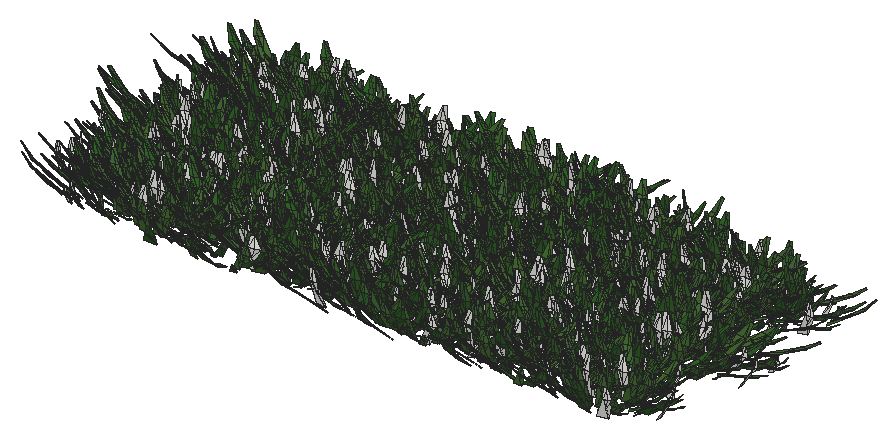
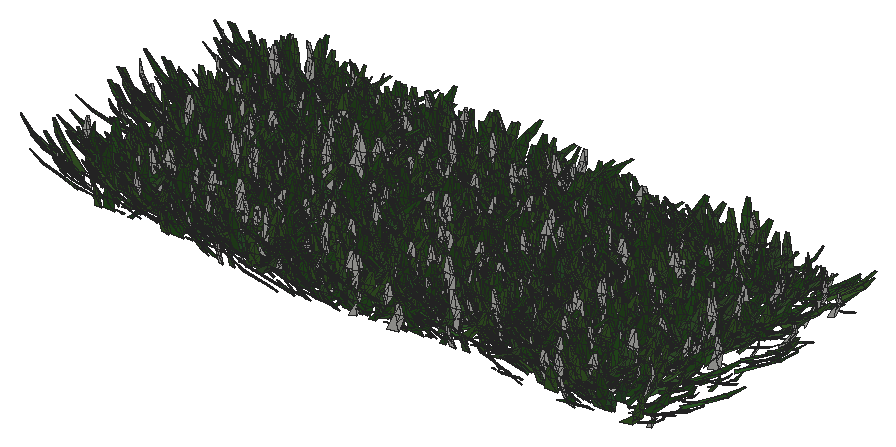
# SketchUp Ruby script. Lengths in inches.
U = 1.inch
M = Sketchup.active_model
def pt(a) = Geom::Point3d.new(a.map { |v| v * U })
def face(e, loops, mat)
  f = e.add_face(loops[0].map { |a| pt(a) })
  loops[1..].each { |l| e.add_face(l.map { |a| pt(a) }).erase! }
  f.material = f.back_material = mat if mat
  f
end
# faces: each face lists its corners as indices into pts; further lists are holes
def faces(e, pts, list, mat = nil) = list.each { |f| face(e, (f[0].is_a?(Array) ? f : [f]).map { |l| l.map { |i| pts[i] } }, mat) }
# xy, xz, yz: faces in a plane at the given z, y or x. An outline is a flat list of corners, or four numbers for a rectangle; further outlines are holes
def ring(l) = l.size == 4 ? [[l[0], l[1]], [l[2], l[1]], [l[2], l[3]], [l[0], l[3]]] : l.each_slice(2).to_a
def flat(e, list, mat, &to3) = list.each { |f| face(e, (f[0].is_a?(Array) ? f : [f]).map { |l| ring(l).map { |u, v| to3.(u, v) } }, mat) }
def xy(e, z, list, mat = nil) = flat(e, list, mat) { |x, y| [x, y, z] }
def xz(e, y, list, mat = nil) = flat(e, list, mat) { |x, z| [x, y, z] }
def yz(e, x, list, mat = nil) = flat(e, list, mat) { |y, z| [x, y, z] }
def lines(e, pts, list) = list.each { |a, b| e.add_line(pt(pts[a]), pt(pts[b])) }
# prism: a flat outline (further loops are holes) pulled along v
def prism(e, loops, v, mat = nil)
  f = face(e, loops, mat); d = Geom::Vector3d.new(v.map { |x| x * U })
  f.pushpull(f.normal.samedirection?(d) ? d.length : -d.length)
end
def box(e, o, s, mat = nil) = prism(e, [[o, [o[0] + s[0], o[1], o[2]], [o[0] + s[0], o[1] + s[1], o[2]], [o[0], o[1] + s[1], o[2]]]], [0, 0, s[2]], mat)
def at(x, y, z, deg = 0) = Geom::Transformation.translation(pt([x, y, z])) * Geom::Transformation.rotation(ORIGIN, Z_AXIS, deg.degrees)
def axes(o, x, y, z) = Geom::Transformation.new([*x, 0, *y, 0, *z, 0, *pt(o).to_a, 1])
def part(name) = M.definitions.add(name)
# library, detail: a bought-in or finely detailed component or shape, given as its bounding box
def library(name, o, s) = part(name).tap { |d| box(d.entities, o, s) }
def detail(e, o, s) = box(e.add_group.entities, o, s)
def put(e, d, t, mat = nil) = e.add_instance(d, t).tap { |i| i.material = mat if mat }
def group(e, t, mat = nil) = e.add_group.tap { |g| g.transformation = t; g.material = mat if mat }.entities
root = M.entities
M.materials.add("Material82").color = [68, 110, 58]
M.materials.add("Material83").color = [48, 90, 38]
M.materials.add("Material84").color = [68, 110, 48]
M.materials.add("Material85").color = [48, 90, 48]
M.materials.add("Material86").color = [58, 110, 58]
M.materials.add("Material87").color = [58, 90, 38]
M.materials.add("Material88").color = [68, 100, 58]
M.materials.add("Material89").color = [48, 100, 38]
c1 = part("grass00")
p = [[-0.6875,0.15,0],[-0.56,0.08,5.52],[-0.04,0.03,2.76],[0.48,-0.02,0],[0.35,-0.02,5.52],[-0.1,-0.14,5.52],
  [-0.12,0.65,8.37],[-0.42,0.65,8.37]]
faces(c1.entities,p,[[0,1,2,3],[3,2,4],[1,5,2],[5,4,2],[1,6,5],[4,5,6],[7,6,1]])
c2 = part("Group16\#1")
put(c2.entities,c1,axes([1.44,-0.61,-0.01],[0.05352,0.12609,0],[-0.10704,0.04543,0.07239],[0.06664,-0.02828,0.11628]),"Material85")
put(c2.entities,c1,axes([0.76,-0.15,-0.01],[0.04676,0.24062,0],[-0.23162,0.04501,0.06642],[0.0652,-0.01267,0.23595]),"Material82")
put(c2.entities,c1,axes([0.79,0.01,-0.01],[-0.00606,0.34651,0],[-0.34381,-0.00602,0.0432],[0.04319,0.00076,0.34386]))
put(c2.entities,c1,axes([1,0.23,-0.01],[-0.07192,0.31144,0],[-0.28722,-0.06632,0.1236],[0.12043,0.02781,0.29478]),"Material84")
put(c2.entities,c1,axes([1.66,0.77,-0.01],[-0.13828,0.29651,0],[-0.21551,-0.1005,0.22471],[0.20365,0.09498,0.23779]),"Material89")
put(c2.entities,c1,axes([0.6875,0.52,-0.01],[-0.18126,0.24051,0],[-0.22746,-0.17142,0.09788],[0.07817,0.05891,0.28481]),"Material84")
put(c2.entities,c1,axes([0.68,0.78,-0.01],[-0.215,0.18688,0],[-0.12385,-0.14248,0.21334],[0.13995,0.16101,0.18878]),"Material82")
put(c2.entities,c1,axes([0.56,1,-0.01],[-0.13756,0.07624,0],[-0.06159,-0.11112,0.0927],[0.04494,0.08108,0.12705]),"Material84")
put(c2.entities,c1,axes([0.2,0.64,-0.01],[-0.23729,0.07254,0],[-0.05711,-0.18681,0.153],[0.04473,0.14632,0.19535]),"Material89")
put(c2.entities,c1,axes([0.0625,0.72,-0.01],[-0.28874,0.02525,0],[-0.02179,-0.24916,0.14647],[0.01276,0.14591,0.25012]),"Material82")
put(c2.entities,c1,axes([-0.08,0.62,-0.01],[-0.34089,-0.04187,0],[0.03255,-0.26504,0.216],[-0.02633,0.21439,0.26703]),"Material89")
put(c2.entities,c1,axes([-0.34,0.98,-0.01],[-0.14314,-0.0493,0],[0.04397,-0.12769,0.06843],[-0.02228,0.0647,0.13505]),"Material89")
put(c2.entities,c1,axes([-0.87,1.45,-0.01],[-0.23488,-0.14114,0],[0.13761,-0.22901,0.06087],[-0.03135,0.05217,0.26717]))
put(c2.entities,c1,axes([-0.72,0.77,-0.01],[-0.14208,-0.13251,0],[0.07209,-0.0773,0.16301],[-0.11118,0.11922,0.1057]),"Material89")
put(c2.entities,c1,axes([-0.62,0.43,-0.01],[-0.14845,-0.21203,0],[0.18654,-0.13061,0.12304],[-0.10079,0.07057,0.22772]),"Material82")
put(c2.entities,c1,axes([-0.68,0.29,-0.01],[-0.13639,-0.32136,0],[0.31723,-0.13464,0.05579],[-0.05136,0.0218,0.34462]),"Material83")
put(c2.entities,c1,axes([-0.64,0.125,-0.01],[-0.0458,-0.23569,0],[0.22124,-0.043,0.08276],[-0.08124,0.01579,0.22538]),"Material86")
put(c2.entities,c1,axes([-1.6,-0.03,-0.01],[0.00576,-0.32897,0],[0.27526,0.00482,0.18018],[-0.18015,-0.00315,0.2753]),"Material84")
put(c2.entities,c1,axes([-1.36,-0.31,-0.01],[0.05718,-0.24765,0],[0.18172,0.04196,0.17267],[-0.16825,-0.03885,0.1865]),"Material89")
put(c2.entities,c1,axes([-1.54,-0.72,-0.01],[0.06537,-0.14017,0],[0.13555,0.06321,0.03939],[-0.0357,-0.01665,0.14956]))
put(c2.entities,c1,axes([-1.19,-0.9,-0.01],[0.09597,-0.12735,0],[0.11214,0.08451,0.07557],[-0.06035,-0.04548,0.14042]),"Material88")
put(c2.entities,c1,axes([-0.47,-0.54,-0.01],[0.11588,-0.10072,0],[0.0618,0.0711,0.12124],[-0.07953,-0.0915,0.0942]))
put(c2.entities,c1,axes([-0.47,-0.84,-0.01],[0.11927,-0.0661,0],[0.06603,0.11913,0.00646],[-0.00313,-0.00565,0.13621]),"Material84")
put(c2.entities,c1,axes([-0.38,-1.24,-0.01],[0.28037,-0.08571,0],[0.0618,0.20215,0.20315],[-0.05939,-0.19428,0.21139]),"Material88")
put(c2.entities,c1,axes([-0.06,-0.66,-0.01],[0.22719,-0.01987,0],[0.01247,0.14255,0.17758],[-0.01547,-0.17691,0.1431]),"Material87")
put(c2.entities,c1,axes([0.11,-0.89,-0.01],[0.14882,0.01828,0],[-0.01058,0.08611,0.12229],[0.01491,-0.12138,0.08676]),"Material85")
put(c2.entities,c1,axes([0.25,-0.72,-0.01],[0.20481,0.07053,0],[-0.06206,0.18022,0.10291],[0.03351,-0.0973,0.1906]),"Material85")
put(c2.entities,c1,axes([0.85,-1.42,-0.01],[0.16481,0.09904,0],[-0.09472,0.15762,0.05616],[0.02893,-0.04814,0.18389]),"Material84")
put(c2.entities,c1,axes([1.01,-1.09,-0.01],[0.21858,0.20385,0],[-0.17495,0.1876,0.15339],[0.10462,-0.11218,0.25652]),"Material89")
put(c2.entities,c1,axes([1.01,-0.71,-0.01],[0.08733,0.12473,0],[-0.06445,0.04512,0.13037],[0.1068,-0.07477,0.07867]),"Material85")
c3 = part("Group15\#1")
put(c3.entities,c2,at(0,0,0))
c4 = part("3darcstudiotree_grass00\#1")
put(c4.entities,c3,at(0,0,0))
put(root,c4,axes([699.52,311.06,-34.17],[4.38861,-0.21228,0],[0.43057,1.38444,-0.03723],[0.02239,0.072,1.30959]))
put(root,c4,axes([685.5,310.76,-34.17],[-4.13743,-0.67569,0],[1.3247,-1.26157,-0.00358],[0.00873,-0.00832,1.65637]))
put(root,c4,axes([708.43,310.87,-34.17],[-4.01536,-0.24387,0],[0.54359,-1.39202,-0.03709],[0.03558,-0.0911,1.68681]))
put(root,c4,axes([689.4,311.1,-34.17],[-2.56412,-1.04956,0],[2.92241,-1.11041,-0.03217],[0.12075,-0.04588,1.58546]))
put(root,c4,axes([666.81,311.63,-34.17],[2.70248,-1.34249,0],[3.67105,1.14936,-0.06314],[0.18316,0.05735,1.30132]))
put(root,c4,axes([657.125,311.57,-34.17],[-0.72323,-1.62263,0],[3.80365,-0.26368,-0.04893],[0.28769,-0.01994,1.72817]))
put(root,c4,axes([663.9,311.85,-34.17],[3.75674,0.29184,0],[-0.86575,1.73332,-0.03192],[-0.02673,0.05352,1.45488]))
put(root,c4,axes([710.66,311.9,-34.17],[-1.60231,-1.37282,0],[3.29691,-0.59848,-0.04546],[0.27162,-0.04931,1.78943]))
put(root,c4,axes([650.6,312.09,-34.17],[2.778,0.72584,0],[-2.53603,1.50959,-0.00365],[-0.00789,0.0047,1.34685]))
put(root,c4,axes([696.92,312.09,-34.17],[-2.06199,-1.44492,0],[3.43124,-0.76156,-0.05229],[0.2544,-0.05646,1.64764]))
put(root,c4,axes([673.79,312.32,-34.17],[3.70563,0.39578,0],[-0.96164,1.40032,-0.0432],[-0.06214,0.09049,1.51727]))
put(root,c4,axes([680.75,311.99,-34.17],[-2.71187,1.03836,0],[-2.98144,-1.21104,-0.01854],[-0.0717,-0.02913,1.78092]))
put(root,c4,axes([673.21,313.2,-34.17],[3.3945,-0.58791,0],[1.6844,1.5126,-0.00525],[0.01109,0.00996,1.64886]))
put(root,c4,axes([652.32,312.94,-34.17],[3.42042,0.9713,0],[-2.12433,1.16348,-0.02682],[-0.10129,0.05548,1.76121]))
put(root,c4,axes([691.01,313.4,-34.17],[-1.338,-1.30891,0],[3.60545,-0.57321,-0.00075],[0.00363,-0.00058,1.52674]))
put(root,c4,axes([683.32,313.55,-34.17],[-3.93883,-1.01936,0],[1.86002,-1.11781,-0.04657],[0.18505,-0.11121,1.84036]))
put(root,c4,axes([711.02,314.01,-34.17],[0.96155,-1.39333,0],[3.31195,0.35548,-0.01758],[0.11319,0.01215,1.71636]))
put(root,c4,axes([705.99,313.53,-34.17],[-0.63419,1.43243,0],[-3.71512,-0.25582,-0.03794],[-0.18856,-0.01298,1.42617]))
put(root,c4,axes([679.27,314.07,-34.17],[-2.9141,-1.11595,0],[2.66035,-1.08046,-0.03796],[0.14613,-0.05935,1.58175]))
put(root,c4,axes([701.39,314.11,-34.17],[-2.17802,-1.23467,0],[3.55396,-0.97507,-0.03629],[0.13271,-0.03641,1.44541]))
put(root,c4,axes([658.15,314.21,-34.17],[-2.20792,-1.57829,0],[3.78019,-0.82247,-0.0117],[0.05427,-0.01181,1.7149]))
put(root,c4,axes([666.23,314.45,-34.17],[0.29138,-1.80133,0],[3.99838,0.10059,-0.05413],[0.25015,0.00629,1.39055]))
put(root,c4,axes([661.49,314.54,-34.17],[4.00255,0.79486,0],[-1.95042,1.52752,-0.03278],[-0.08544,0.06692,1.8841]))
put(root,c4,axes([694.75,314.43,-34.17],[-3.86108,-0.00922,0],[0.0279,-1.817,-0.0591],[0.00158,-0.1028,1.52309]))
put(root,c4,axes([686.01,315.13,-34.17],[-1.35898,-1.3893,0],[3.82798,-0.58237,-0.03571],[0.20852,-0.03172,1.92492]))
put(root,c4,axes([695.74,315.64,-34.17],[-0.67683,-1.69031,0],[4.16932,-0.25965,-0.01303],[0.08012,-0.00499,1.96953]))
put(root,c4,axes([691.02,315.19,-34.17],[-3.01219,1.1686,0],[-2.47695,-0.99299,-0.0233],[-0.1132,-0.04538,1.83382]))
put(root,c4,axes([656.43,315.52,-34.17],[3.87339,1.05779,0],[-2.14052,1.21905,-0.05103],[-0.17397,0.09908,1.6877]))
put(root,c4,axes([663.91,315.8125,-34.17],[-3.28835,-0.7389,0],[1.7462,-1.20864,-0.01205],[0.03007,-0.02081,1.33255]))
put(root,c4,axes([672.49,316.1,-34.17],[3.72756,0.95688,0],[-1.9535,1.18357,-0.02904],[-0.10466,0.06341,1.7729]))
put(root,c4,axes([678.02,316.64,-34.17],[2.31636,-1.46039,0],[3.68995,0.91026,-0.01393],[0.05236,0.01292,1.44657]))
put(root,c4,axes([667.04,316.43,-34.17],[4.20535,0.69684,0],[-1.48182,1.39084,-0.00848],[-0.02193,0.02058,1.91304]))
put(root,c4,axes([708.75,316.58,-34.17],[3.11027,0.45791,0],[-1.48719,1.57105,-0.03179],[-0.06172,0.0652,1.76952]))
put(root,c4,axes([651.74,316.37,-34.17],[-3.34476,-0.15722,0],[0.48645,-1.60959,-0.01308],[0.00826,-0.02735,1.64432]))
put(root,c4,axes([701.39,316.43,-34.17],[-1.50877,1.48911,0],[-3.61563,-0.56976,-0.0529],[-0.26655,-0.042,1.58349]))
put(root,c4,axes([678.79,317.29,-34.17],[1.60686,-1.51832,0],[3.56667,0.58707,-0.05171],[0.27066,0.04455,1.64301]))
put(root,c4,axes([666.78,317.89,-34.17],[3.97377,-0.0043,0],[0.0116,1.66593,-0.02008],[0.00028,0.04042,1.61638]))
put(root,c4,axes([657.68,317.88,-34.17],[-0.75362,-1.53541,0],[3.24661,-0.24784,-0.00678],[0.04146,-0.00316,1.54322]))
put(root,c4,axes([684.59,317.61,-34.17],[-1.22945,1.37189,0],[-3.12548,-0.43563,-0.03966],[-0.20868,-0.02909,1.38647]))
put(root,c4,axes([696.96,317.54,-34.17],[-2.26778,1.36387,0],[-3.7802,-0.97758,-0.05216],[-0.16857,-0.04359,1.30947]))
put(root,c4,axes([700.9,318.68,-34.17],[3.45505,-0.2676,0],[0.73895,1.48387,-0.00241],[0.00289,0.0058,1.79003]))
put(root,c4,axes([705.54,318.27,-34.17],[-3.53984,-0.54558,0],[1.35048,-1.36277,-0.02269],[0.0488,-0.04924,1.64292]))
put(root,c4,axes([664.04,318.51,-34.17],[2.55644,1.08061,0],[-3.46336,1.27432,-0.03325],[-0.10953,0.0403,1.59934]))
put(root,c4,axes([690.76,318.18,-34.17],[-0.71352,1.56405,0],[-4.14814,-0.29432,-0.02584],[-0.10481,-0.00744,1.30174]))
put(root,c4,axes([650.01,318.26,-34.17],[-0.26231,1.84263,0],[-3.30675,-0.07321,-0.00552],[-0.03272,-0.00072,1.47331]))
put(root,c4,axes([672.46,318.43,-34.17],[0.91997,1.29984,0],[-3.25818,0.35865,-0.02635],[-0.1448,0.01594,1.4463]))
put(root,c4,axes([673.37,319.7,-34.17],[3.30024,-0.68967,0],[2.06464,1.53659,-0.00115],[0.00232,0.00173,1.42878]))
put(root,c4,axes([682.92,320.24,-34.17],[2.55399,-1.11237,0],[2.83561,1.01258,-0.04299],[0.17745,0.06336,1.59659]))
put(root,c4,axes([651.875,320.08,-34.17],[3.21897,1.19921,0],[-3.23164,1.34914,-0.01632],[-0.04651,0.01942,1.46423]))
put(root,c4,axes([664.26,319.8,-34.17],[-0.44896,1.44211,0],[-4.03082,-0.19517,-0.03564],[-0.19872,-0.00962,1.71014]))
put(root,c4,axes([696.96,319.67,-34.17],[-1.84352,1.61201,0],[-4.26993,-0.75947,-0.03185],[-0.15055,-0.02678,1.82087]))
put(root,c4,axes([680.86,319.98,-34.17],[-3.29654,-0.72222,0],[2.17338,-1.54289,-0.02959],[0.0707,-0.05019,1.65043]))
put(root,c4,axes([656.62,320.74,-34.17],[1.85229,-1.14191,0],[3.43107,0.86561,-0.02581],[0.11483,0.02897,1.61243]))
put(root,c4,axes([666.45,320.76,-34.17],[0.37581,-1.33084,0],[4.05324,0.17801,-0.00391],[0.01773,0.00078,1.39627]))
put(root,c4,axes([690.49,321.01,-34.17],[3.4977,-1.17788,0],[2.34178,1.08154,-0.01134],[0.04108,0.01897,1.5074]))
put(root,c4,axes([701.44,320.44,-34.17],[-2.729,0.78907,0],[-2.0311,-1.09252,-0.03589],[-0.15909,-0.08558,1.93035]))
put(root,c4,axes([707.34,320.46,-34.17],[-2.28466,1.61729,0],[-3.8326,-0.84205,-0.0557],[-0.22938,-0.0504,1.55009]))
put(root,c4,axes([708.74,321.7,-34.17],[1.96831,-1.06776,0],[3.09361,0.88694,-0.02782],[0.14847,0.04257,1.89124]))
put(root,c4,axes([694.53,321.65,-34.17],[0.83797,-1.39271,0],[3.20742,0.30015,-0.04624],[0.35526,0.03324,1.95114]))
put(root,c4,axes([692.51,321.81,-34.17],[3.50844,-0.55754,0],[1.25662,1.22985,-0.02314],[0.04614,0.04516,1.34449]))
put(root,c4,axes([649.65,321.85,-34.17],[3.19452,-0.59612,0],[1.46474,1.2208,-0.01286],[0.03129,0.02608,1.45976]))
put(root,c4,axes([711.52,321.67,-34.17],[-1.71956,-1.37213,0],[4.12265,-0.80354,-0.04891],[0.23955,-0.04669,1.88309]))
put(root,c4,axes([655.95,321.92,-34.17],[0.90068,-1.41561,0],[4.53027,0.44829,-0.03647],[0.13709,0.01357,1.35653]))
put(root,c4,axes([661.22,321.66,-34.17],[-2.78639,1.08314,0],[-3.04744,-1.21928,-0.00446],[-0.01393,-0.00557,1.44777]))
put(root,c4,axes([673.35,322.33,-34.17],[-2.22834,-1.37792,0],[3.47538,-0.87412,-0.04256],[0.18098,-0.04552,1.55835]))
put(root,c4,axes([700.6,322.67,-34.17],[-3.88555,-0.79581,0],[2.02489,-1.53765,-0.03725],[0.08107,-0.06156,1.55507]))
put(root,c4,axes([681.28,322.68,-34.17],[-4.41332,-0.66754,0],[1.63018,-1.67623,-0.02874],[0.04038,-0.04152,1.33872]))
put(root,c4,axes([669.94,322.74,-34.17],[-3.79387,-0.48377,0],[1.38418,-1.6883,-0.04655],[0.0671,-0.08184,1.58019]))
put(root,c4,axes([683.77,322.64,-34.17],[-4.27576,-0.00967,0],[0.01971,-1.35519,-0.00073],[0.00002,-0.00168,1.50826]))
put(root,c4,axes([691.92,324.16,-34.17],[1.98892,-1.13086,0],[3.89758,1.06614,-0.02169],[0.07891,0.02158,1.57389]))
put(root,c4,axes([668.61,324.52,-34.17],[2.33801,-1.27151,0],[3.45385,0.98774,-0.00976],[0.0468,0.01338,1.89325]))
put(root,c4,axes([708.62,324.23,-34.17],[-3.20918,-1.37059,0],[3.45166,-1.25697,-0.04946],[0.15315,-0.05577,1.48426]))
put(root,c4,axes([661.91,324.53,-34.17],[3.64852,0.24315,0],[-0.61045,1.42466,-0.04218],[-0.04748,0.11082,1.85529]))
put(root,c4,axes([652.32,324.15,-34.17],[-2.66899,1.32243,0],[-3.00544,-0.94339,-0.02078],[-0.10429,-0.03273,1.84714]))
put(root,c4,axes([656.21,324.96,-34.17],[4.17155,-0.17702,0],[0.50263,1.84221,-0.03237],[0.01504,0.05512,1.52951]))
put(root,c4,axes([695.49,324.84,-34.17],[2.88531,0.9286,0],[-2.55752,1.23593,-0.03119],[-0.12387,0.05986,1.90467]))
put(root,c4,axes([683.125,324.58,-34.17],[-2.10798,1.40451,0],[-3.51427,-0.82033,-0.03668],[-0.20421,-0.04767,1.98009]))
put(root,c4,axes([679.27,324.83,-34.17],[1.47468,1.38827,0],[-3.83437,0.63347,-0.03717],[-0.17802,0.02941,1.61797]))
put(root,c4,axes([711.1,324.8,-34.17],[0.13535,1.36053,0],[-4.14262,0.0641,-0.00595],[-0.03791,0.00059,1.98232]))
put(root,c4,axes([672.11,324.7,-34.17],[-3.1837,0.9292,0],[-2.49148,-1.32767,-0.01624],[-0.05606,-0.02987,1.82169]))
put(root,c4,axes([702.23,325.44,-34.17],[-4.08688,-0.61044,0],[1.62889,-1.6961,-0.00084],[0.00115,-0.0012,1.34285]))
put(root,c4,axes([694.73,326.12,-34.17],[1.67099,-1.73753,0],[3.10475,0.46439,-0.00605],[0.0444,0.00664,1.95327]))
put(root,c4,axes([651.42,326.34,-34.17],[4.2125,0.29861,0],[-0.756,1.65872,-0.00017],[-0.00017,0.00037,1.78268]))
put(root,c4,axes([679.04,326.29,-34.17],[4.05845,0.38101,0],[-1.01694,1.68476,-0.06215],[-0.0714,0.11828,1.63292]))
put(root,c4,axes([706.13,326.37,-34.17],[-1.7024,-1.44396,0],[3.0538,-0.55996,-0.04244],[0.29035,-0.05324,1.90455]))
put(root,c4,axes([668.9375,326.42,-34.17],[-0.84806,-1.31842,0],[3.86352,-0.38651,-0.05601],[0.32758,-0.03277,1.80254]))
put(root,c4,axes([664.03,326.47,-34.17],[-2.64127,-0.90818,0],[2.55598,-1.15614,-0.03875],[0.14904,-0.06742,1.70607]))
put(root,c4,axes([683.96,326.41,-34.17],[-3.43779,0.5694,0],[-1.45981,-1.37078,-0.01995],[-0.04437,-0.04166,1.62326]))
put(root,c4,axes([658.91,326.62,-34.17],[-2.26233,1.10327,0],[-2.6855,-0.85647,-0.00747],[-0.03039,-0.00969,1.35493]))
put(root,c4,axes([712.21,326.58,-34.17],[-3.44248,1.19972,0],[-2.84327,-1.26888,-0.04086],[-0.12277,-0.05479,1.46035]))
put(root,c4,axes([688.95,327.37,-34.17],[3.38923,-0.39007,0],[1.26949,1.71555,-0.04654],[0.05157,0.06969,1.34343]))
put(root,c4,axes([672.92,327.55,-34.17],[-1.79663,-1.22383,0],[3.52148,-0.80403,-0.02105],[0.11606,-0.0265,1.94345]))
put(root,c4,axes([703.375,327.4375,-34.17],[-4.21718,-0.04667,0],[0.09647,-1.35575,-0.03959],[0.00846,-0.11883,1.96257]))
put(root,c4,axes([662.62,328.35,-34.17],[-3.15245,-0.45856,0],[1.56973,-1.67838,-0.02933],[0.05139,-0.05494,1.72129]))
put(root,c4,axes([699.56,328.42,-34.17],[1.70731,1.1244,0],[-2.88773,0.68196,-0.04808],[-0.30467,0.07195,1.86326]))
put(root,c4,axes([706.56,328.375,-34.17],[-2.99752,0.92431,0],[-2.30263,-1.1614,-0.02144],[-0.09164,-0.04622,1.94421]))
put(root,c4,axes([677.7,328.69,-34.17],[-0.05283,1.30539,0],[-4.56112,-0.02871,-0.04794],[-0.23084,-0.00145,1.64652]))
put(root,c4,axes([651.84,328.75,-34.17],[-4.04939,0.05434,0],[-0.15117,-1.75202,-0.01213],[-0.00231,-0.02678,1.86653]))
put(root,c4,axes([697.67,329.47,-34.17],[3.97524,-0.29729,0],[0.87691,1.8237,-0.05959],[0.04913,0.10217,1.56123]))
put(root,c4,axes([669.16,329.22,-34.17],[4.25696,0.81021,0],[-1.71809,1.40397,-0.05424],[-0.1086,0.08874,1.36476]))
put(root,c4,axes([672.89,328.85,-34.17],[-2.04292,1.4828,0],[-3.7482,-0.80316,-0.0267],[-0.09668,-0.02072,1.31753]))
put(root,c4,axes([682.99,329.62,-34.17],[3.62862,0.35052,0],[-1.11939,1.8023,-0.01455],[-0.01942,0.03128,1.97892]))
put(root,c4,axes([657.32,329.82,-34.17],[2.6006,-1.2072,0],[3.21281,1.07644,-0.02612],[0.11842,0.03968,1.8801]))
put(root,c4,axes([689.01,329.65,-34.17],[-3.56945,0.98002,0],[-2.54129,-1.43957,-0.02528],[-0.0766,-0.04339,1.76765]))
put(root,c4,axes([673.47,330.68,-34.17],[0.7854,-1.46662,0],[3.6757,0.30614,-0.00249],[0.01359,0.00113,1.57305]))
put(root,c4,axes([692.42,330.8125,-34.17],[1.68218,-1.47179,0],[3.03421,0.53937,-0.02223],[0.13236,0.02353,1.62899]))
put(root,c4,axes([700.87,330.9375,-34.17],[0.3333,-1.68825,0],[3.84573,0.11808,-0.01871],[0.11577,0.00355,1.79426]))
put(root,c4,axes([663.06,330.71,-34.17],[3.57061,0.64267,0],[-1.40632,1.21522,-0.03533],[-0.10777,0.09312,1.86502]))
put(root,c4,axes([650.66,330.5625,-34.17],[-2.58541,-0.85496,0],[2.80483,-1.31917,-0.0116],[0.03194,-0.01502,1.40225]))
put(root,c4,axes([708.24,331.1,-34.17],[3.17331,-0.50017,0],[1.66687,1.64477,-0.02256],[0.03879,0.03827,1.55958]))
put(root,c4,axes([668.5625,330.6,-34.17],[-3.33443,-0.23634,0],[0.70723,-1.55188,-0.01818],[0.01451,-0.03184,1.35222]))
put(root,c4,axes([679.93,331.65,-34.17],[-1.63027,-1.73131,0],[4.11958,-0.60332,-0.00006],[0.00033,-0.00005,1.81412]))
put(root,c4,axes([694.52,331.4,-34.17],[-2.03219,1.40442,0],[-2.95743,-0.66557,-0.04437],[-0.22116,-0.04977,1.46464]))
put(root,c4,axes([659.04,331.75,-34.17],[0.61227,1.37165,0],[-4.42146,0.30696,-0.06022],[-0.31422,0.02181,1.78296]))
put(root,c4,axes([684.93,331.97,-34.17],[1.42302,1.52353,0],[-4.19442,0.60932,-0.04046],[-0.17686,0.02569,1.56076]))
put(root,c4,axes([686.92,332.93,-34.17],[3.4755,-0.56156,0],[1.30477,1.25594,-0.00746],[0.01674,0.01612,1.52751]))
put(root,c4,axes([662.67,332.83,-34.17],[-1.74555,-1.44076,0],[3.95857,-0.74592,-0.00689],[0.03295,-0.00621,1.74288]))
put(root,c4,axes([703.54,332.7,-34.17],[-0.75802,1.26839,0],[-3.28645,-0.30547,-0.04738],[-0.26314,-0.02446,1.4441]))
put(root,c4,axes([691.6875,333.17,-34.17],[-1.97999,-1.67359,0],[3.87039,-0.71217,-0.01753],[0.07436,-0.01368,1.49864]))
put(root,c4,axes([697.79,332.85,-34.17],[0.81482,1.77329,0],[-4.44159,0.31742,-0.02342],[-0.11628,0.00831,1.70718]))
put(root,c4,axes([678.3,332.92,-34.17],[0.46872,1.37145,0],[-4.27579,0.22728,-0.05207],[-0.28533,0.01517,1.7882]))
put(root,c4,axes([710.54,332.8,-34.17],[-1.06746,1.42925,0],[-3.87706,-0.45036,-0.01201],[-0.05554,-0.00645,1.46096]))
put(root,c4,axes([672.13,333.8,-34.17],[3.33835,-0.04276,0],[0.15045,1.82678,-0.05593],[0.00839,0.10182,1.60461]))
put(root,c4,axes([706.83,333.75,-34.17],[-0.95803,-1.53129,0],[3.44538,-0.33525,-0.01268],[0.07432,-0.00723,1.60602]))
put(root,c4,axes([666.75,333.9,-34.17],[0.3233,-1.61244,0],[3.70268,0.11546,-0.00365],[0.02017,0.00063,1.54435]))
put(root,c4,axes([656.86,333.31,-34.17],[-3.72731,0.81099,0],[-1.84954,-1.32207,-0.01481],[-0.0358,-0.02559,1.43556]))
put(root,c4,axes([653.57,333.43,-34.17],[-1.62678,1.3546,0],[-3.70168,-0.6914,-0.05633],[-0.31213,-0.0583,1.88219]))
put(root,c4,axes([707.35,335.17,-34.17],[0.20206,-1.72347,0],[4.27325,0.07792,-0.04434],[0.21389,0.0039,1.54852]))
put(root,c4,axes([655.84,335.47,-34.17],[1.41685,-1.43454,0],[3.76136,0.57778,-0.0174],[0.0698,0.01072,1.30214]))
put(root,c4,axes([652.35,334.875,-34.17],[-3.91283,-0.66077,0],[1.78522,-1.64415,-0.00601],[0.01088,-0.01002,1.5624]))
put(root,c4,axes([711.76,335.08,-34.17],[-3.8816,-0.56323,0],[1.5517,-1.6632,-0.01333],[0.02356,-0.02525,1.7245]))
put(root,c4,axes([688.68,335.43,-34.17],[3.63174,0.64343,0],[-1.49454,1.312,-0.04301],[-0.1083,0.09507,1.6797]))
put(root,c4,axes([661,335.92,-34.17],[-1.36397,-1.5291,0],[3.40561,-0.47247,-0.03242],[0.15123,-0.02098,1.33794]))
put(root,c4,axes([699.81,335.38,-34.17],[-2.70631,1.45447,0],[-3.636,-1.05223,-0.06171],[-0.25363,-0.0734,1.72322]))
put(root,c4,axes([684.61,335.71,-34.17],[1.95907,1.41788,0],[-3.34699,0.71925,-0.025],[-0.15312,0.03291,1.99255]))
put(root,c4,axes([673.95,336.08,-34.17],[-0.62966,-1.28695,0],[4.54348,-0.34574,-0.02161],[0.1197,-0.00911,1.95654]))
put(root,c4,axes([666.34,335.76,-34.17],[-3.55761,-0.37183,0],[0.9234,-1.37408,-0.01321],[0.02436,-0.03625,1.9444]))
put(root,c4,axes([696.62,335.77,-34.17],[-1.83042,1.58988,0],[-3.0568,-0.54735,-0.0444],[-0.26156,-0.04683,1.62807]))
put(root,c4,axes([678.07,336.05,-34.17],[-3.95397,0.70682,0],[-1.69994,-1.479,-0.00714],[-0.01245,-0.01084,1.30481]))
put(root,c4,axes([661.35,337.1,-34.17],[4.34464,0.20061,0],[-0.52956,1.78372,-0.02723],[-0.01491,0.05022,1.60719]))
put(root,c4,axes([656.54,337.02,-34.17],[1.20267,1.27774,0],[-3.21983,0.47135,-0.04291],[-0.22552,0.03301,1.44315]))
put(root,c4,axes([694.82,338.01,-34.17],[1.32812,-1.21732,0],[3.65511,0.62022,-0.02985],[0.14197,0.02409,1.54439]))
put(root,c4,axes([668.24,337.8,-34.17],[-1.97159,-1.316,0],[4.00038,-0.93213,-0.05519],[0.24758,-0.05769,1.81465]))
put(root,c4,axes([651.34,337.59,-34.17],[-4.26775,-0.24104,0],[0.59342,-1.63411,-0.00988],[0.00789,-0.02172,1.76639]))
put(root,c4,axes([702.43,337.4375,-34.17],[-3.54904,1.16368,0],[-2.54993,-1.20953,-0.00935],[-0.03236,-0.01535,1.61847]))
put(root,c4,axes([689.03,337.55,-34.17],[-3.22115,0.33319,0],[-1.15137,-1.73117,-0.03948],[-0.04657,-0.07003,1.58152]))
put(root,c4,axes([705.12,337.82,-34.17],[-3.58911,0.17625,0],[-0.41421,-1.31187,-0.03309],[-0.02615,-0.08283,1.60704]))
put(root,c4,axes([711.08,337.73,-34.17],[-3.46015,1.06405,0],[-2.06953,-1.04669,-0.02241],[-0.08068,-0.04081,1.47722]))
put(root,c4,axes([672.8,337.8,-34.17],[-3.47223,1.22215,0],[-3.01377,-1.3317,-0.01139],[-0.0395,-0.01745,1.76647]))
put(root,c4,axes([683.36,337.97,-34.17],[-1.73682,1.47733,0],[-4.1333,-0.75577,-0.04346],[-0.21523,-0.03935,1.86413]))
put(root,c4,axes([678.08,338.51,-34.17],[-0.9909,1.30306,0],[-3.23471,-0.38257,-0.04553],[-0.22482,-0.02659,1.30482]))
put(root,c4,axes([694.65,339.13,-34.17],[-1.94812,-1.05267,0],[3.13916,-0.90354,-0.00015],[0.00082,-0.00024,1.94435]))
put(root,c4,axes([650.62,339.66,-34.17],[2.46062,-1.19689,0],[3.08233,0.98555,-0.02965],[0.1062,0.03396,1.3715]))
put(root,c4,axes([657.16,339.35,-34.17],[-0.1961,1.67231,0],[-3.9427,-0.07191,-0.00948],[-0.04368,-0.0008,1.36423]))
put(root,c4,axes([680.125,339.77,-34.17],[4.39717,0.52423,0],[-1.00944,1.31686,-0.04581],[-0.07981,0.10411,1.57403]))
put(root,c4,axes([684.58,340.18,-34.17],[3.00521,0.63807,0],[-1.62064,1.18715,-0.02125],[-0.05194,0.03805,1.32121]))
